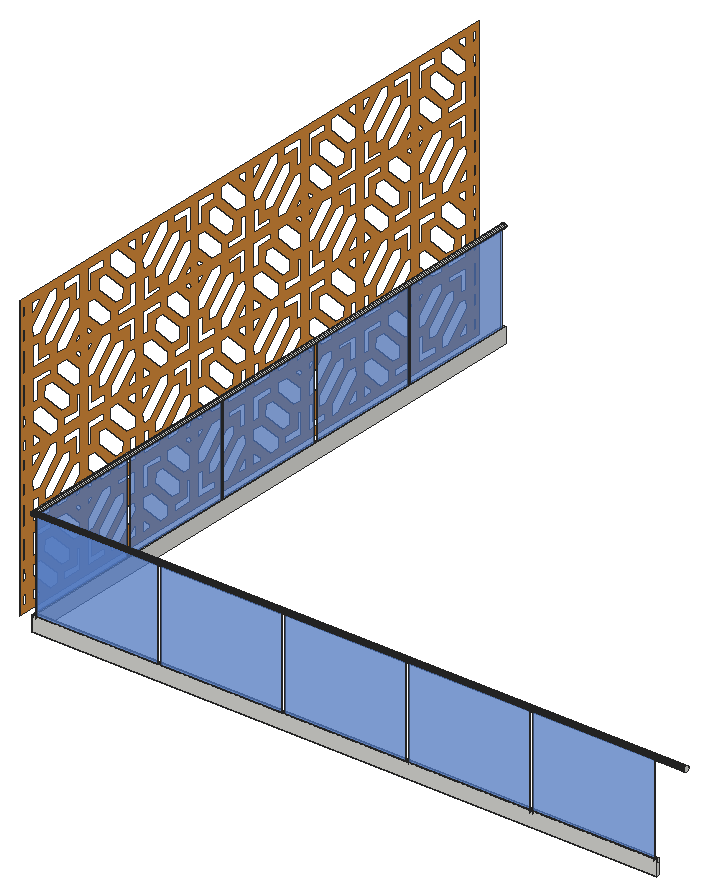
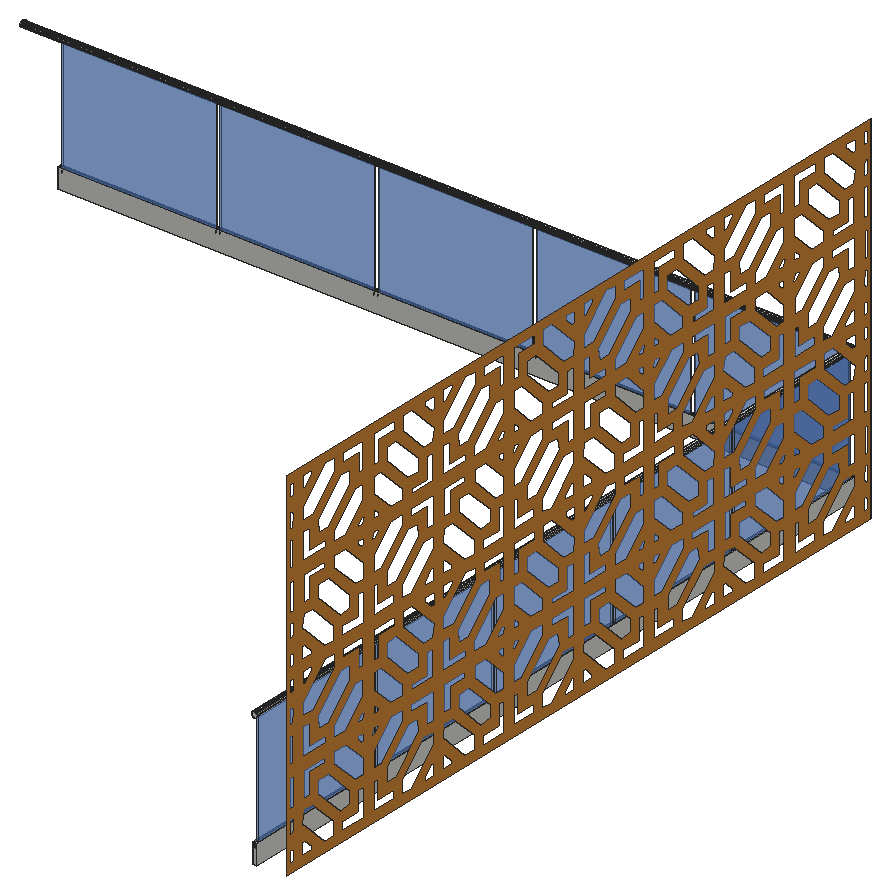
# SketchUp Ruby script. Lengths in inches.
U = 1.inch
M = Sketchup.active_model
def pt(a) = Geom::Point3d.new(a.map { |v| v * U })
def face(e, loops, mat)
  f = e.add_face(loops[0].map { |a| pt(a) })
  loops[1..].each { |l| e.add_face(l.map { |a| pt(a) }).erase! }
  f.material = f.back_material = mat if mat
  f
end
# faces: each face lists its corners as indices into pts; further lists are holes
def faces(e, pts, list, mat = nil) = list.each { |f| face(e, (f[0].is_a?(Array) ? f : [f]).map { |l| l.map { |i| pts[i] } }, mat) }
# xy, xz, yz: faces in a plane at the given z, y or x. An outline is a flat list of corners, or four numbers for a rectangle; further outlines are holes
def ring(l) = l.size == 4 ? [[l[0], l[1]], [l[2], l[1]], [l[2], l[3]], [l[0], l[3]]] : l.each_slice(2).to_a
def flat(e, list, mat, &to3) = list.each { |f| face(e, (f[0].is_a?(Array) ? f : [f]).map { |l| ring(l).map { |u, v| to3.(u, v) } }, mat) }
def xy(e, z, list, mat = nil) = flat(e, list, mat) { |x, y| [x, y, z] }
def xz(e, y, list, mat = nil) = flat(e, list, mat) { |x, z| [x, y, z] }
def yz(e, x, list, mat = nil) = flat(e, list, mat) { |y, z| [x, y, z] }
def lines(e, pts, list) = list.each { |a, b| e.add_line(pt(pts[a]), pt(pts[b])) }
# prism: a flat outline (further loops are holes) pulled along v
def prism(e, loops, v, mat = nil)
  f = face(e, loops, mat); d = Geom::Vector3d.new(v.map { |x| x * U })
  f.pushpull(f.normal.samedirection?(d) ? d.length : -d.length)
end
def box(e, o, s, mat = nil) = prism(e, [[o, [o[0] + s[0], o[1], o[2]], [o[0] + s[0], o[1] + s[1], o[2]], [o[0], o[1] + s[1], o[2]]]], [0, 0, s[2]], mat)
def at(x, y, z, deg = 0) = Geom::Transformation.translation(pt([x, y, z])) * Geom::Transformation.rotation(ORIGIN, Z_AXIS, deg.degrees)
def axes(o, x, y, z) = Geom::Transformation.new([*x, 0, *y, 0, *z, 0, *pt(o).to_a, 1])
def part(name) = M.definitions.add(name)
# library, detail: a bought-in or finely detailed component or shape, given as its bounding box
def library(name, o, s) = part(name).tap { |d| box(d.entities, o, s) }
def detail(e, o, s) = box(e.add_group.entities, o, s)
def put(e, d, t, mat = nil) = e.add_instance(d, t).tap { |i| i.material = mat if mat }
def group(e, t, mat = nil) = e.add_group.tap { |g| g.transformation = t; g.material = mat if mat }.entities
root = M.entities
M.materials.add("1056 AP 9903 Mellow Melon-N").color = [219, 142, 59]
M.materials.add("[Translucent Glass Blue]").color = [100, 149, 237]
M.materials["[Translucent Glass Blue]"].alpha = 0.5
c1 = part("Glass Rail Spacer")
box(c1.entities,[-0.5,-0.25,0],[1,0.5,1])
c2 = part("Group48\#2")
xz(c2.entities,0,[[0.01,0,-0.18,0.02,-0.37,0.09,-0.52,0.21,-0.64,0.37,-0.72,0.54,-0.75,0.74,-0.73,0.93,-0.66,1.12,-0.54,1.27,-0.38,1.39,-0.21,1.47,-0.01,1.5,0.18,1.48,0.37,1.41,0.52,1.29,0.64,1.13,0.72,0.96,0.75,0.76,0.73,0.57,0.66,0.38,0.54,0.23,0.38,0.11,0.21,0.03]])
yz(c2.entities,214.51,[[-193.11,0,-192.92,0.03,-192.74,0.11,-192.59,0.23,-192.47,0.38,-192.4,0.57,-192.375,0.76,-192.4,0.96,-192.48,1.13,-192.6,1.29,-192.76,1.41,-192.94,1.48,-193.14,1.5,-193.33,1.47,-193.51,1.39,-193.66,1.27,-193.78,1.12,-193.85,0.93,-193.875,0.74,-193.85,0.54,-193.77,0.37,-193.65,0.21,-193.49,0.09,-193.31,0.02]])
p = [[-0.18,0,0.02],[-0.18,-193.31,0.02],[-0.37,-193.49,0.09],[-0.37,0,0.09],[214.51,-193.31,0.02],[214.51,-193.49,0.09],
  [0.01,0,0],[0.01,-193.11,0],[214.51,-193.11,0],[0.21,0,0.03],[0.21,-192.92,0.03],[214.51,-192.92,0.03],
  [0.38,0,0.11],[0.38,-192.74,0.11],[214.51,-192.74,0.11],[-0.52,-193.65,0.21],[-0.52,0,0.21],[214.51,-193.65,0.21],
  [0.54,0,0.23],[0.54,-192.59,0.23],[214.51,-192.59,0.23],[-0.64,-193.77,0.37],[-0.64,0,0.37],[214.51,-193.77,0.37],
  [0.66,0,0.38],[0.66,-192.47,0.38],[214.51,-192.47,0.38],[-0.72,-193.85,0.54],[-0.72,0,0.54],[214.51,-193.85,0.54],
  [0.73,0,0.57],[0.73,-192.4,0.57],[214.51,-192.4,0.57],[-0.75,-193.875,0.74],[-0.75,0,0.74],[214.51,-193.875,0.74],
  [0.75,0,0.76],[0.75,-192.375,0.76],[214.51,-192.375,0.76],[-0.73,-193.85,0.93],[-0.73,0,0.93],[214.51,-193.85,0.93],
  [0.72,0,0.96],[0.72,-192.4,0.96],[214.51,-192.4,0.96],[-0.66,-193.78,1.12],[-0.66,0,1.12],[214.51,-193.78,1.12],
  [0.64,0,1.13],[0.64,-192.48,1.13],[214.51,-192.48,1.13],[-0.54,-193.66,1.27],[-0.54,0,1.27],[214.51,-193.66,1.27],
  [0.52,0,1.29],[0.52,-192.6,1.29],[214.51,-192.6,1.29],[-0.38,-193.51,1.39],[-0.38,0,1.39],[214.51,-193.51,1.39],
  [0.37,0,1.41],[0.37,-192.76,1.41],[214.51,-192.76,1.41],[-0.21,-193.33,1.47],[-0.21,0,1.47],[214.51,-193.33,1.47],
  [0.18,0,1.48],[0.18,-192.94,1.48],[214.51,-192.94,1.48],[-0.01,-193.14,1.5],[-0.01,0,1.5],[214.51,-193.14,1.5]]
faces(c2.entities,p,[[0,1,2,3],[1,4,5,2],[6,7,1,0],[7,8,4,1],[9,10,7,6],[10,11,8,7],[12,13,10,9],[13,14,11,10],
  [3,2,15,16],[2,5,17,15],[18,19,13,12],[19,20,14,13],[16,15,21,22],[15,17,23,21],[24,25,19,18],[25,26,20,19],
  [22,21,27,28],[21,23,29,27],[30,31,25,24],[31,32,26,25],[28,27,33,34],[27,29,35,33],[36,37,31,30],[37,38,32,31],
  [34,33,39,40],[33,35,41,39],[42,43,37,36],[43,44,38,37],[40,39,45,46],[39,41,47,45],[48,49,43,42],[49,50,44,43],
  [46,45,51,52],[45,47,53,51],[54,55,49,48],[55,56,50,49],[52,51,57,58],[51,53,59,57],[60,61,55,54],[61,62,56,55],
  [58,57,63,64],[57,59,65,63],[66,67,61,60],[67,68,62,61],[64,63,69,70],[63,65,71,69],[70,69,67,66],[69,71,68,67]])
c3 = part("Group51\#1")
xy(c3.entities,0,[[-0.5,-193.625,-0.5,0,0.5,0,0.5,-192.625],[-0.5,-193.625,0.5,-192.625,205.08,-192.625,205.08,-193.625]])
xy(c3.entities,4,[[-0.25,-193.375,0.25,-192.875,0.25,0,-0.25,0],[-0.25,-193.375,205.08,-193.375,205.08,-192.875,0.25,-192.875]])
xy(c3.entities,5,[[-0.5,-193.625,-0.25,-193.375,-0.25,0,-0.5,0],[-0.5,-193.625,205.08,-193.625,205.08,-193.375,-0.25,-193.375],[0.25,-192.875,0.5,-192.625,0.5,0,0.25,0],[0.25,-192.875,205.08,-192.875,205.08,-192.625,0.5,-192.625]])
xz(c3.entities,-193.625,[[-0.5,0,205.08,5]])
xz(c3.entities,-193.375,[[-0.25,4,205.08,5]])
xz(c3.entities,-192.875,[[0.25,4,205.08,5]])
xz(c3.entities,-192.625,[[0.5,0,205.08,5]])
xz(c3.entities,0,[[-0.5,0,-0.5,5,-0.25,5,-0.25,4,0.25,4,0.25,5,0.5,5,0.5,0]])
yz(c3.entities,-0.5,[[-193.625,0,0,5]])
yz(c3.entities,-0.25,[[-193.375,4,0,5]])
yz(c3.entities,0.25,[[-192.875,4,0,5]])
yz(c3.entities,0.5,[[-192.625,0,0,5]])
yz(c3.entities,205.08,[[-193.625,0,-192.625,0,-192.625,5,-192.875,5,-192.875,4,-193.375,4,-193.375,5,-193.625,5]])
c4 = part("Group52\#1")
box(c4.entities,[-0.1875,0,0],[0.375,37.48,30])
c5 = part("Group53\#1")
box(c5.entities,[-0.1875,0,0],[0.375,37.48,30])
c6 = part("Group54\#1")
box(c6.entities,[-0.1875,0,0],[0.375,37.48,30])
c7 = part("Group55\#1")
box(c7.entities,[-0.1875,0,0],[0.375,37.47,30])
c8 = part("Group56\#1")
box(c8.entities,[-0.1875,0,0],[0.375,37.47,30])
c9 = part("Group57\#1")
box(c9.entities,[-0.1875,0,0],[0.375,39.87,30],"[Translucent Glass Blue]")
c10 = part("Group58\#1")
box(c10.entities,[-0.1875,0,0],[0.375,39.87,30])
c11 = part("Group59\#1")
box(c11.entities,[-0.1875,0,0],[0.375,39.87,30])
c12 = part("Group60\#1")
box(c12.entities,[-0.1875,0,0],[0.375,39.87,30])
c13 = part("Group61\#1")
box(c13.entities,[-0.1875,0,0],[0.375,39.87,30])
c14 = part("Glass Railing\#1")
put(c14.entities,c1,at(0,0,4,-90))
put(c14.entities,c1,at(0,-38.48,4,-90))
put(c14.entities,c1,at(0,-76.95,4,-90))
put(c14.entities,c1,at(0,-115.43,4,-90))
put(c14.entities,c1,at(0,-153.9,4,-90))
put(c14.entities,c1,at(0,-192.375,4,-90))
put(c14.entities,c1,at(0.25,-192.625,4))
put(c14.entities,c1,at(41.12,-192.625,4))
put(c14.entities,c1,at(81.98,-192.625,4))
put(c14.entities,c1,at(122.85,-192.625,4))
put(c14.entities,c1,at(163.72,-192.625,4))
put(c14.entities,c1,at(204.58,-192.625,4))
put(c14.entities,c2,at(0,0.5,34))
put(c14.entities,c3,at(0,0.5,0))
put(c14.entities,c4,at(0,-0.5,4,180),"[Translucent Glass Blue]")
put(c14.entities,c5,at(0,-38.98,4,180),"[Translucent Glass Blue]")
put(c14.entities,c6,at(0,-77.45,4,180),"[Translucent Glass Blue]")
put(c14.entities,c7,at(0,-115.93,4,180),"[Translucent Glass Blue]")
put(c14.entities,c8,at(0,-154.4,4,180),"[Translucent Glass Blue]")
put(c14.entities,c9,at(0.75,-192.625,4,-90))
put(c14.entities,c10,at(41.62,-192.625,4,-90),"[Translucent Glass Blue]")
put(c14.entities,c11,at(82.48,-192.625,4,-90),"[Translucent Glass Blue]")
put(c14.entities,c12,at(123.35,-192.625,4,-90),"[Translucent Glass Blue]")
put(c14.entities,c13,at(164.22,-192.625,4,-90),"[Translucent Glass Blue]")
yz(root,15.0625,[[[13.79,145.75,202.3125,238.4375],[94.27,153.04,91.29,153.47,91.29,156.53,98.2,163.43,101.6,163.43,101.6,160.37],[94.27,198.38,91.29,198.8125,91.29,201.875,98.2,208.78,101.6,208.78,101.6,205.71],[69.15,220.75,69.15,223.82,76.48,231.15,79.46,230.72,79.46,227.66,72.56,220.75],[23.81,175.41,23.81,178.47,31.14,185.81,34.12,185.375,34.12,182.3125,27.21,175.41],[23.81,220.75,23.81,223.82,31.14,231.15,34.12,230.72,34.12,227.66,27.21,220.75],[69.15,175.41,69.15,178.47,76.48,185.81,79.46,185.375,79.46,182.3125,72.56,175.41],[159.84,220.75,159.84,223.82,167.17,231.15,170.15,230.72,170.15,227.66,163.24,220.75],[159.84,175.41,159.84,178.47,167.17,185.81,170.15,185.375,170.15,182.3125,163.24,175.41],[48.93,153.04,45.95,153.47,45.95,156.53,52.85,163.43,56.26,163.43,56.26,160.37],[48.93,198.38,45.95,198.8125,45.95,201.875,52.85,208.78,56.26,208.78,56.26,205.71],[139.62,153.04,136.64,153.47,136.64,156.53,143.54,163.43,146.95,163.43,146.95,160.37],[184.96,153.04,181.98,153.47,181.98,156.53,188.88,163.43,192.29,163.43,192.29,160.37],[184.96,198.38,181.98,198.8125,181.98,201.875,188.88,208.78,192.29,208.78,192.29,205.71],[139.62,198.38,136.64,198.8125,136.64,201.875,143.54,208.78,146.95,208.78,146.95,205.71],[114.49,220.75,114.49,223.82,121.83,231.15,124.81,230.72,124.81,227.66,117.9,220.75],[114.49,175.41,114.49,178.47,121.83,185.81,124.81,185.375,124.81,182.3125,117.9,175.41],[98.27,175.34,91.36,182.24,91.36,185.65,94.43,185.65,101.76,178.32,101.33,175.34],[98.27,220.68,91.36,227.59,91.36,230.99,94.43,230.99,101.76,223.66,101.33,220.68],[52.92,175.34,46.02,182.24,46.02,185.65,49.09,185.65,56.42,178.32,55.99,175.34],[30.98,198.54,23.65,205.87,24.08,208.85,27.14,208.85,34.05,201.95,34.05,198.54],[76.32,198.54,68.99,205.87,69.42,208.85,72.49,208.85,79.39,201.95,79.39,198.54],[143.61,175.34,136.71,182.24,136.71,185.65,139.77,185.65,147.1,178.32,146.68,175.34],[52.92,220.68,46.02,227.59,46.02,230.99,49.09,230.99,56.42,223.66,55.99,220.68],[76.32,153.19,68.99,160.53,69.42,163.51,72.49,163.51,79.39,156.6,79.39,153.19],[30.98,153.19,23.65,160.53,24.08,163.51,27.14,163.51,34.05,156.6,34.05,153.19],[143.61,220.68,136.71,227.59,136.71,230.99,139.77,230.99,147.1,223.66,146.68,220.68],[121.67,198.54,114.34,205.87,114.77,208.85,117.83,208.85,124.73,201.95,124.73,198.54],[167.01,198.54,159.68,205.87,160.11,208.85,163.17,208.85,170.08,201.95,170.08,198.54],[188.96,175.34,182.05,182.24,182.05,185.65,185.12,185.65,192.45,178.32,192.02,175.34],[188.96,220.68,182.05,227.59,182.05,230.99,185.12,230.99,192.45,223.66,192.02,220.68],[121.67,153.19,114.34,160.53,114.77,163.51,117.83,163.51,124.73,156.6,124.73,153.19],[167.01,153.19,159.68,160.53,160.11,163.51,163.17,163.51,170.08,156.6,170.08,153.19],[96.45,148.27,96.45,151.76,103.35,158.67,106.33,158.67,106.76,155.61,99.42,148.27],[141.79,148.27,141.79,151.76,148.7,158.67,151.67,158.67,152.11,155.61,144.77,148.27],[96.45,193.61,96.45,197.11,103.35,204.01,106.33,204.01,106.76,200.95,99.42,193.61],[141.79,193.61,141.79,197.11,148.7,204.01,151.67,204.01,152.11,200.95,144.77,193.61],[187.14,148.27,187.14,151.76,194.04,158.67,197.02,158.67,197.45,155.61,190.11,148.27],[51.11,148.27,51.11,151.76,58.01,158.67,60.99,158.67,61.42,155.61,54.08,148.27],[187.14,193.61,187.14,197.11,194.04,204.01,197.02,204.01,197.45,200.95,190.11,193.61],[51.11,193.61,51.11,197.11,58.01,204.01,60.99,204.01,61.42,200.95,54.08,193.61],[193.72,225.84,186.82,232.74,186.82,235.72,189.88,236.15,197.22,228.8125,197.22,225.84],[193.72,180.49,186.82,187.4,186.82,190.375,189.88,190.81,197.22,183.47,197.22,180.49],[26.22,193.38,18.88,200.72,18.88,203.69,22.375,203.69,29.28,196.79,29.28,193.8125],[71.5625,193.38,64.22,200.72,64.22,203.69,67.72,203.69,74.625,196.79,74.625,193.8125],[116.91,193.38,109.57,200.72,109.57,203.69,113.0625,203.69,119.97,196.79,119.97,193.8125],[162.25,193.38,154.91,200.72,154.91,203.69,158.41,203.69,165.3125,196.79,165.3125,193.8125],[26.22,148.03,18.88,155.375,18.88,158.35,22.375,158.35,29.28,151.45,29.28,148.47],[71.5625,148.03,64.22,155.375,64.22,158.35,67.72,158.35,74.625,151.45,74.625,148.47],[116.91,148.03,109.57,155.375,109.57,158.35,113.0625,158.35,119.97,151.45,119.97,148.47],[162.25,148.03,154.91,155.375,154.91,158.35,158.41,158.35,165.3125,151.45,165.3125,148.47],[103.04,225.84,96.13,232.74,96.13,235.72,99.19,236.15,106.53,228.8125,106.53,225.84],[103.04,180.49,96.13,187.4,96.13,190.375,99.19,190.81,106.53,183.47,106.53,180.49],[148.38,225.84,141.48,232.74,141.48,235.72,144.54,236.15,151.875,228.8125,151.875,225.84],[148.38,180.49,141.48,187.4,141.48,190.375,144.54,190.81,151.875,183.47,151.875,180.49],[57.69,225.84,50.79,232.74,50.79,235.72,53.85,236.15,61.1875,228.8125,61.1875,225.84],[57.69,180.49,50.79,187.4,50.79,190.375,53.85,190.81,61.1875,183.47,61.1875,180.49],[109.77,225.52,109.33,228.58,116.67,235.92,119.65,235.92,119.65,232.42,112.75,225.52],[109.77,180.18,109.33,183.24,116.67,190.58,119.65,190.58,119.65,187.08,112.75,180.18],[155.11,225.52,154.68,228.58,162.02,235.92,164.99,235.92,164.99,232.42,158.09,225.52],[155.11,180.18,154.68,183.24,162.02,190.58,164.99,190.58,164.99,187.08,158.09,180.18],[64.42,180.18,63.99,183.24,71.33,190.58,74.31,190.58,74.31,187.08,67.4,180.18],[64.42,225.52,63.99,228.58,71.33,235.92,74.31,235.92,74.31,232.42,67.4,225.52],[19.08,225.52,18.65,228.58,25.99,235.92,28.96,235.92,28.96,232.42,22.06,225.52],[19.08,180.18,18.65,183.24,25.99,190.58,28.96,190.58,28.96,187.08,22.06,180.18],[28.96,216.42,28.96,219.05,35.87,225.95,38.41,225.95,38.41,222.03,32.8,216.42],[74.31,216.42,74.31,219.05,81.21,225.95,83.76,225.95,83.76,222.03,78.15,216.42],[28.96,171.08,28.96,173.71,35.87,180.61,38.41,180.61,38.41,176.68,32.8,171.08],[74.31,171.08,74.31,173.71,81.21,180.61,83.76,180.61,83.76,176.68,78.15,171.08],[119.65,216.42,119.65,219.05,126.55,225.95,129.1,225.95,129.1,222.03,123.49,216.42],[164.99,216.42,164.99,219.05,171.9,225.95,174.45,225.95,174.45,222.03,168.84,216.42],[119.65,171.08,119.65,173.71,126.55,180.61,129.1,180.61,129.1,176.68,123.49,171.08],[164.99,171.08,164.99,173.71,171.9,180.61,174.45,180.61,174.45,176.68,168.84,171.08],[183.33,216.39,177.72,221.99,177.72,225.84,180.35,225.84,187.25,218.93,187.25,216.39],[92.64,216.39,87.03,221.99,87.03,225.84,89.66,225.84,96.56,218.93,96.56,216.39],[47.3,216.39,41.6875,221.99,41.6875,225.84,44.32,225.84,51.22,218.93,51.22,216.39],[137.98,216.39,132.375,221.99,132.375,225.84,135,225.84,141.91,218.93,141.91,216.39],[183.33,171.04,177.72,176.65,177.72,180.49,180.35,180.49,187.25,173.59,187.25,171.04],[92.64,171.04,87.03,176.65,87.03,180.49,89.66,180.49,96.56,173.59,96.56,171.04],[47.3,171.04,41.6875,176.65,41.6875,180.49,44.32,180.49,51.22,173.59,51.22,171.04],[137.98,171.04,132.375,176.65,132.375,180.49,135,180.49,141.91,173.59,141.91,171.04],[35.75,203.69,28.85,210.6,28.85,213.15,32.77,213.15,38.38,207.54,38.38,203.69],[35.75,158.35,28.85,165.25,28.85,167.8,32.77,167.8,38.38,162.19,38.38,158.35],[81.09,203.69,74.19,210.6,74.19,213.15,78.11,213.15,83.72,207.54,83.72,203.69],[171.78,203.69,164.88,210.6,164.88,213.15,168.8,213.15,174.41,207.54,174.41,203.69],[81.09,158.35,74.19,165.25,74.19,167.8,78.11,167.8,83.72,162.19,83.72,158.35],[126.4375,203.69,119.53,210.6,119.53,213.15,123.46,213.15,129.07,207.54,129.07,203.69],[171.78,158.35,164.88,165.25,164.88,167.8,168.8,167.8,174.41,162.19,174.41,158.35],[126.4375,158.35,119.53,165.25,119.53,167.8,123.46,167.8,129.07,162.19,129.07,158.35],[132.34,203.58,132.34,207.5,137.95,213.11,141.79,213.11,141.79,210.48,134.89,203.58],[132.34,158.23,132.34,162.16,137.95,167.77,141.79,167.77,141.79,165.14,134.89,158.23],[87,203.58,87,207.5,92.61,213.11,96.45,213.11,96.45,210.48,89.54,203.58],[41.65,203.58,41.65,207.5,47.26,213.11,51.11,213.11,51.11,210.48,44.2,203.58],[41.65,158.23,41.65,162.16,47.26,167.77,51.11,167.77,51.11,165.14,44.2,158.23],[177.68,203.58,177.68,207.5,183.29,213.11,187.14,213.11,187.14,210.48,180.23,203.58],[87,158.23,87,162.16,92.61,167.77,96.45,167.77,96.45,165.14,89.54,158.23],[177.68,158.23,177.68,162.16,183.29,167.77,187.14,167.77,187.14,165.14,180.23,158.23],[132.34,148.27,132.34,155.63,134.06,155.63,134.06,150.43,139.21,150.43,139.21,148.27],[132.34,193.61,132.34,200.98,134.06,200.98,134.06,195.78,139.21,195.78,139.21,193.61],[36.7,183.21,36.7,188.41,31.54,188.41,31.54,190.58,38.41,190.58,38.41,183.21],[87,148.27,87,155.63,88.72,155.63,88.72,150.43,93.87,150.43,93.87,148.27],[172.73,183.21,172.73,188.41,167.57,188.41,167.57,190.58,174.45,190.58,174.45,183.21],[177.68,148.27,177.68,155.63,179.4,155.63,179.4,150.43,184.56,150.43,184.56,148.27],[87,193.61,87,200.98,88.72,200.98,88.72,195.78,93.87,195.78,93.87,193.61],[36.7,228.55,36.7,233.75,31.54,233.75,31.54,235.92,38.41,235.92,38.41,228.55],[82.04,183.21,82.04,188.41,76.88,188.41,76.88,190.58,83.76,190.58,83.76,183.21],[41.65,148.27,41.65,155.63,43.37,155.63,43.37,150.43,48.53,150.43,48.53,148.27],[177.68,193.61,177.68,200.98,179.4,200.98,179.4,195.78,184.56,195.78,184.56,193.61],[172.73,228.55,172.73,233.75,167.57,233.75,167.57,235.92,174.45,235.92,174.45,228.55],[41.65,193.61,41.65,200.98,43.37,200.98,43.37,195.78,48.53,195.78,48.53,193.61],[82.04,228.55,82.04,233.75,76.88,233.75,76.88,235.92,83.76,235.92,83.76,228.55],[127.38,183.21,127.38,188.41,122.23,188.41,122.23,190.58,129.1,190.58,129.1,183.21],[127.38,228.55,127.38,233.75,122.23,233.75,122.23,235.92,129.1,235.92,129.1,228.55],[189.85,216.39,189.85,218.1,195.05,218.1,195.05,223.26,197.22,223.26,197.22,216.39],[109.57,206.27,109.57,213.15,116.93,213.15,116.93,211.43,111.73,211.43,111.73,206.27],[99.16,216.39,99.16,218.1,104.37,218.1,104.37,223.26,106.53,223.26,106.53,216.39],[144.51,216.39,144.51,218.1,149.71,218.1,149.71,223.26,151.875,223.26,151.875,216.39],[53.82,216.39,53.82,218.1,59.02,218.1,59.02,223.26,61.1875,223.26,61.1875,216.39],[154.91,206.27,154.91,213.15,162.28,213.15,162.28,211.43,157.08,211.43,157.08,206.27],[189.85,171.04,189.85,172.76,195.05,172.76,195.05,177.92,197.22,177.92,197.22,171.04],[109.57,160.93,109.57,167.8,116.93,167.8,116.93,166.08,111.73,166.08,111.73,160.93],[99.16,171.04,99.16,172.76,104.37,172.76,104.37,177.92,106.53,177.92,106.53,171.04],[144.51,171.04,144.51,172.76,149.71,172.76,149.71,177.92,151.875,177.92,151.875,171.04],[53.82,171.04,53.82,172.76,59.02,172.76,59.02,177.92,61.1875,177.92,61.1875,171.04],[154.91,160.93,154.91,167.8,162.28,167.8,162.28,166.08,157.08,166.08,157.08,160.93],[18.88,206.27,18.88,213.15,26.25,213.15,26.25,211.43,21.05,211.43,21.05,206.27],[64.22,206.27,64.22,213.15,71.59,213.15,71.59,211.43,66.39,211.43,66.39,206.27],[64.22,160.93,64.22,167.8,71.59,167.8,71.59,166.08,66.39,166.08,66.39,160.93],[18.88,160.93,18.88,167.8,26.25,167.8,26.25,166.08,21.05,166.08,21.05,160.93],[31.88,193.8125,31.88,195.96,37.08,195.96,37.08,200.6875,38.38,200.6875,38.38,193.8125],[31.88,148.47,31.88,150.62,37.08,150.62,37.08,155.34,38.38,155.34,38.38,148.47],[87.03,183.5,87.03,190.375,93.53,190.375,93.53,188.23,88.33,188.23,88.33,183.5],[77.22,193.8125,77.22,195.96,82.42,195.96,82.42,200.6875,83.72,200.6875,83.72,193.8125],[77.22,148.47,77.22,150.62,82.42,150.62,82.42,155.34,83.72,155.34,83.72,148.47],[87.03,228.84,87.03,235.72,93.53,235.72,93.53,233.57,88.33,233.57,88.33,228.84],[41.6875,183.5,41.6875,190.375,48.1875,190.375,48.1875,188.23,42.99,188.23,42.99,183.5],[41.6875,228.84,41.6875,235.72,48.1875,235.72,48.1875,233.57,42.99,233.57,42.99,228.84],[177.72,183.5,177.72,190.375,184.22,190.375,184.22,188.23,179.02,188.23,179.02,183.5],[132.375,183.5,132.375,190.375,138.875,190.375,138.875,188.23,133.67,188.23,133.67,183.5],[132.375,228.84,132.375,235.72,138.875,235.72,138.875,233.57,133.67,233.57,133.67,228.84],[122.57,148.47,122.57,150.62,127.77,150.62,127.77,155.34,129.07,155.34,129.07,148.47],[122.57,193.8125,122.57,195.96,127.77,195.96,127.77,200.6875,129.07,200.6875,129.07,193.8125],[167.91,193.8125,167.91,195.96,173.11,195.96,173.11,200.6875,174.41,200.6875,174.41,193.8125],[167.91,148.47,167.91,150.62,173.11,150.62,173.11,155.34,174.41,155.34,174.41,148.47],[177.72,228.84,177.72,235.72,184.22,235.72,184.22,233.57,179.02,233.57,179.02,228.84],[194.87,206.61,194.87,211.8125,190.14,211.8125,190.14,213.11,197.02,213.11,197.02,206.61],[19.08,216.42,19.08,222.92,21.23,222.92,21.23,217.72,25.95,217.72,25.95,216.42],[194.87,161.27,194.87,166.47,190.14,166.47,190.14,167.77,197.02,167.77,197.02,161.27],[104.18,206.61,104.18,211.8125,99.46,211.8125,99.46,213.11,106.33,213.11,106.33,206.61],[19.08,171.08,19.08,177.58,21.23,177.58,21.23,172.375,25.95,172.375,25.95,171.08],[109.77,216.42,109.77,222.92,111.92,222.92,111.92,217.72,116.64,217.72,116.64,216.42],[155.11,216.42,155.11,222.92,157.26,222.92,157.26,217.72,161.99,217.72,161.99,216.42],[104.18,161.27,104.18,166.47,99.46,166.47,99.46,167.77,106.33,167.77,106.33,161.27],[64.42,216.42,64.42,222.92,66.57,222.92,66.57,217.72,71.3,217.72,71.3,216.42],[58.84,206.61,58.84,211.8125,54.11,211.8125,54.11,213.11,60.99,213.11,60.99,206.61],[149.53,206.61,149.53,211.8125,144.8,211.8125,144.8,213.11,151.67,213.11,151.67,206.61],[109.77,171.08,109.77,177.58,111.92,177.58,111.92,172.375,116.64,172.375,116.64,171.08],[155.11,171.08,155.11,177.58,157.26,177.58,157.26,172.375,161.99,172.375,161.99,171.08],[58.84,161.27,58.84,166.47,54.11,166.47,54.11,167.77,60.99,167.77,60.99,161.27],[64.42,171.08,64.42,177.58,66.57,177.58,66.57,172.375,71.3,172.375,71.3,171.08],[149.53,161.27,149.53,166.47,144.8,166.47,144.8,167.77,151.67,167.77,151.67,161.27],[200.25,206.27,201.3125,213.15],[200.25,160.93,201.3125,167.8],[14.79,216.39,15.84,223.26],[14.79,171.04,15.84,177.92],[58.41,148.27,58.41,149.14,60.57,151.3,61.42,151.3,61.42,148.27],[58.41,193.61,58.41,194.49,60.57,196.64,61.42,196.64,61.42,193.61],[194.44,148.27,194.44,149.14,196.6,151.3,197.45,151.3,197.45,148.27],[103.75,148.27,103.75,149.14,105.91,151.3,106.76,151.3,106.76,148.27],[149.1,148.27,149.1,149.14,151.25,151.3,152.1,151.3,152.1,148.27],[149.1,193.61,149.1,194.49,151.25,196.64,152.1,196.64,152.1,193.61],[103.75,193.61,103.75,194.49,105.91,196.64,106.76,196.64,106.76,193.61],[194.44,193.61,194.44,194.49,196.6,196.64,197.45,196.64,197.45,193.61],[18.88,193.38,18.88,196.39,19.75,196.39,21.91,194.23,21.91,193.38],[64.22,193.38,64.22,196.39,65.1,196.39,67.26,194.23,67.26,193.38],[109.57,193.38,109.57,196.39,110.44,196.39,112.6,194.23,112.6,193.38],[154.91,193.38,154.91,196.39,155.79,196.39,157.94,194.23,157.94,193.38],[64.22,148.04,64.22,151.05,65.1,151.05,67.26,148.89,67.26,148.04],[18.88,148.04,18.88,151.05,19.75,151.05,21.91,148.89,21.91,148.04],[109.57,148.04,109.57,151.05,110.44,151.05,112.6,148.89,112.6,148.04],[154.91,148.04,154.91,151.05,155.79,151.05,157.94,148.89,157.94,148.04],[196.34,233.14,194.1875,235.3,194.1875,236.15,197.22,236.15,197.22,233.14],[196.34,187.8,194.1875,189.95,194.1875,190.8,197.22,190.8,197.22,187.8],[151,233.14,148.84,235.3,148.84,236.15,151.875,236.15,151.875,233.14],[151,187.8,148.84,189.95,148.84,190.8,151.875,190.8,151.875,187.8],[105.66,233.14,103.5,235.3,103.5,236.15,106.53,236.15,106.53,233.14],[105.66,187.8,103.5,189.95,103.5,190.8,106.53,190.8,106.53,187.8],[60.3125,233.14,58.15,235.3,58.15,236.15,61.1875,236.15,61.1875,233.14],[60.3125,187.8,58.15,189.95,58.15,190.8,61.1875,190.8,61.1875,187.8],[63.99,232.89,63.99,235.92,67,235.92,67,235.04,64.84,232.89],[63.99,187.54,63.99,190.58,67,190.58,67,189.7,64.84,187.54],[109.34,232.89,109.34,235.92,112.35,235.92,112.35,235.04,110.1875,232.89],[109.34,187.54,109.34,190.58,112.35,190.58,112.35,189.7,110.1875,187.54],[154.68,232.89,154.68,235.92,157.6875,235.92,157.6875,235.04,155.53,232.89],[154.68,187.54,154.68,190.58,157.6875,190.58,157.6875,189.7,155.53,187.54],[18.65,232.89,18.65,235.92,21.66,235.92,21.66,235.04,19.5,232.89],[18.65,187.54,18.65,190.58,21.66,190.58,21.66,189.7,19.5,187.54],[200.46,216.42,201.3125,222.92],[200.46,171.08,201.3125,177.58],[14.79,206.61,15.64,213.11],[14.79,161.27,15.64,167.77],[200.46,180.18,200.02,183.24,201.3125,184.53,201.3125,180.18],[200.46,225.52,200.02,228.58,201.3125,229.87,201.3125,225.52],[14.79,154.31,14.79,158.67,15.64,158.67,16.08,155.61],[14.79,199.66,14.79,204.01,15.64,204.01,16.08,200.95],[14.79,148.27,14.79,150.86,15.22,151.3,16.07,151.3,16.07,148.27],[14.79,193.61,14.79,196.21,15.22,196.64,16.07,196.64,16.07,193.61],[200.03,187.54,200.03,190.58,201.3125,190.58,201.3125,187.98,200.875,187.54],[200.03,232.89,200.03,235.92,201.3125,235.92,201.3125,233.32,200.875,232.89],[201.3125,199.66,200.25,200.72,200.25,203.69,201.3125,203.69],[201.3125,154.31,200.25,155.375,200.25,158.35,201.3125,158.35],[14.79,225.84,14.79,229.87,15.84,228.8125,15.84,225.84],[14.79,180.49,14.79,184.53,15.84,183.47,15.84,180.49],[14.97,233.14,14.79,233.32,14.79,236.15,15.84,236.15,15.84,233.14],[14.97,187.8,14.79,187.98,14.79,190.8,15.84,190.8,15.84,187.8],[200.25,193.38,200.25,196.39,201.13,196.39,201.3125,196.21,201.3125,193.38],[200.25,148.04,200.25,151.05,201.13,151.05,201.3125,150.86,201.3125,148.04],[172.73,215.99,172.73,216.86,174.02,218.15,174.45,218.15,174.45,216.42],[36.7,215.99,36.7,216.86,37.99,218.15,38.41,218.15,38.41,216.42],[36.7,170.64,36.7,171.51,37.99,172.81,38.41,172.81,38.41,171.08],[172.73,170.64,172.73,171.51,174.02,172.81,174.45,172.81,174.45,171.08],[82.04,215.99,82.04,216.86,83.33,218.15,83.76,218.15,83.76,216.42],[82.04,170.64,82.04,171.51,83.33,172.81,83.76,172.81,83.76,171.08],[127.38,215.99,127.38,216.86,128.68,218.15,129.1,218.15,129.1,216.42],[127.38,170.64,127.38,171.51,128.68,172.81,129.1,172.81,129.1,171.08],[177.72,216.39,177.28,218.1,178.16,218.1,179.45,216.81,179.45,216.39],[41.6875,216.39,41.25,218.1,42.125,218.1,43.42,216.81,43.42,216.39],[37.94,211.43,36.65,212.72,36.65,213.15,38.38,213.15,38.8125,211.43],[132.375,216.39,131.94,218.1,132.8125,218.1,134.11,216.81,134.11,216.39],[83.29,211.43,81.99,212.72,81.99,213.15,83.72,213.15,84.16,211.43],[173.97,211.43,172.68,212.72,172.68,213.15,174.41,213.15,174.84,211.43],[87.03,216.39,86.6,218.1,87.47,218.1,88.76,216.81,88.76,216.39],[41.6875,171.04,41.25,172.76,42.125,172.76,43.42,171.47,43.42,171.04],[177.72,171.04,177.28,172.76,178.16,172.76,179.45,171.47,179.45,171.04],[128.63,211.43,127.33,212.72,127.33,213.15,129.07,213.15,129.5,211.43],[37.94,166.08,36.65,167.38,36.65,167.8,38.38,167.8,38.8125,166.08],[132.375,171.04,131.94,172.76,132.8125,172.76,134.11,171.47,134.11,171.04],[173.97,166.08,172.68,167.38,172.68,167.8,174.41,167.8,174.84,166.08],[83.29,166.08,81.99,167.38,81.99,167.8,83.72,167.8,84.16,166.08],[87.03,171.04,86.6,172.76,87.47,172.76,88.76,171.47,88.76,171.04],[128.63,166.08,127.33,167.38,127.33,167.8,129.07,167.8,129.5,166.08],[132.34,211.38,132.34,213.11,134.06,213.55,134.06,212.67,132.76,211.38],[177.68,211.38,177.68,213.11,179.4,213.55,179.4,212.67,178.11,211.38],[132.34,166.04,132.34,167.77,134.06,168.2,134.06,167.33,132.76,166.04],[177.68,166.04,177.68,167.77,179.4,168.2,179.4,167.33,178.11,166.04],[87,211.38,87,213.11,88.72,213.55,88.72,212.67,87.42,211.38],[41.65,211.38,41.65,213.11,43.37,213.55,43.37,212.67,42.08,211.38],[87,166.04,87,167.77,88.72,168.2,88.72,167.33,87.42,166.04],[41.65,166.04,41.65,167.77,43.37,168.2,43.37,167.33,42.08,166.04]]],"1056 AP 9903 Mellow Melon-N")
p = [[15.0625,13.79,238.4375],[15.0625,13.79,145.75]]
lines(root,p,[[0,1]])
put(root,c14,at(23.08,202.3125,145.75))
